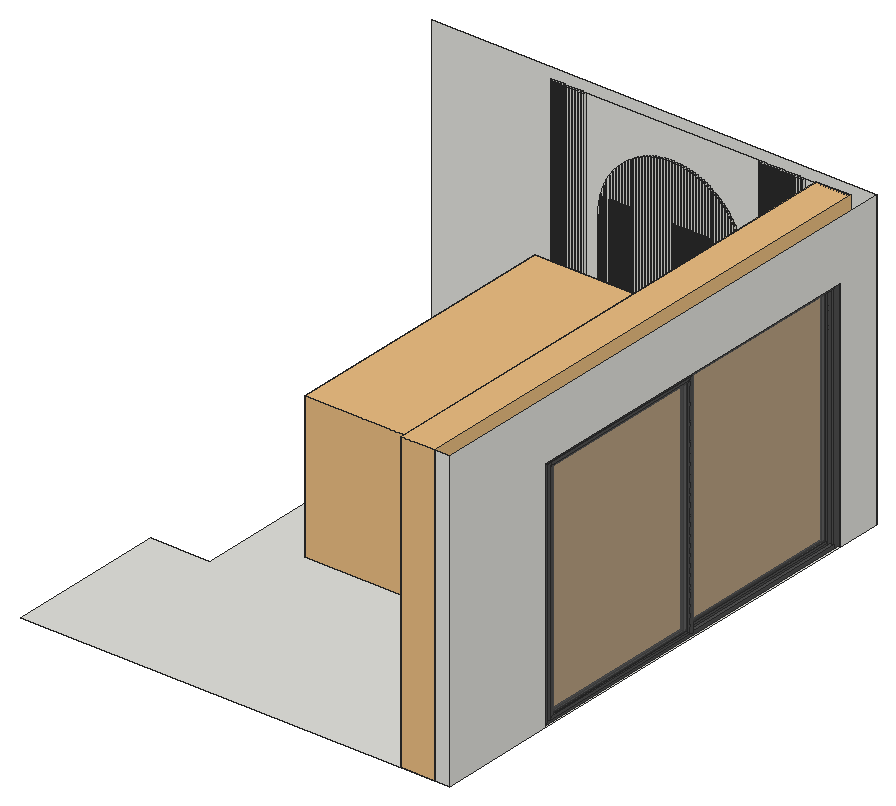
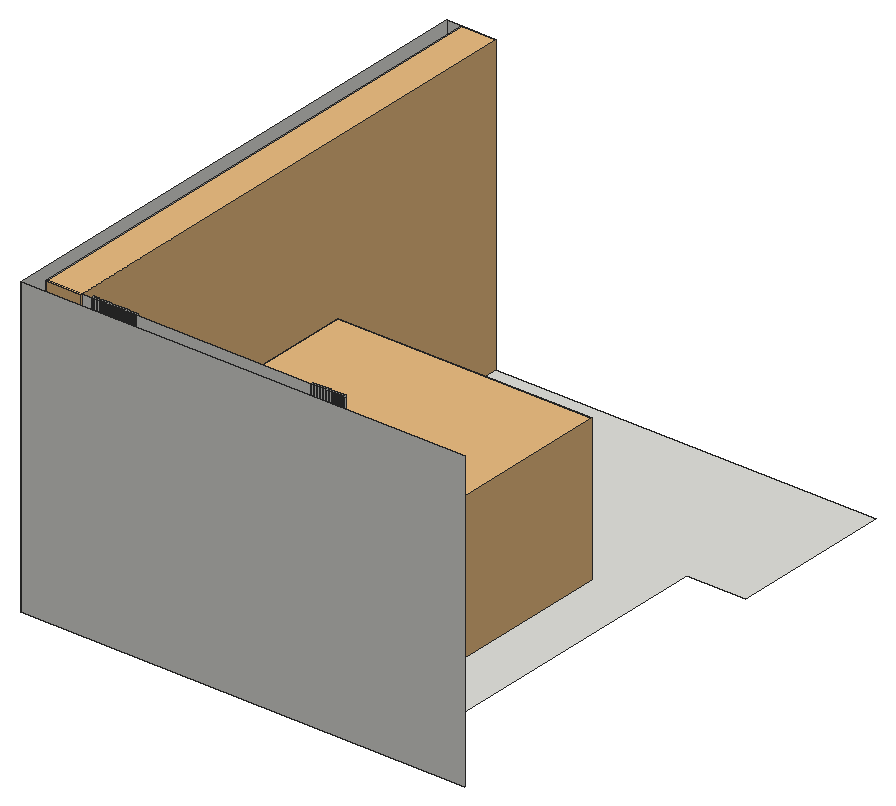
# SketchUp Ruby script. Lengths in inches.
U = 1.inch
M = Sketchup.active_model
def pt(a) = Geom::Point3d.new(a.map { |v| v * U })
def face(e, loops, mat)
  f = e.add_face(loops[0].map { |a| pt(a) })
  loops[1..].each { |l| e.add_face(l.map { |a| pt(a) }).erase! }
  f.material = f.back_material = mat if mat
  f
end
# faces: each face lists its corners as indices into pts; further lists are holes
def faces(e, pts, list, mat = nil) = list.each { |f| face(e, (f[0].is_a?(Array) ? f : [f]).map { |l| l.map { |i| pts[i] } }, mat) }
# xy, xz, yz: faces in a plane at the given z, y or x. An outline is a flat list of corners, or four numbers for a rectangle; further outlines are holes
def ring(l) = l.size == 4 ? [[l[0], l[1]], [l[2], l[1]], [l[2], l[3]], [l[0], l[3]]] : l.each_slice(2).to_a
def flat(e, list, mat, &to3) = list.each { |f| face(e, (f[0].is_a?(Array) ? f : [f]).map { |l| ring(l).map { |u, v| to3.(u, v) } }, mat) }
def xy(e, z, list, mat = nil) = flat(e, list, mat) { |x, y| [x, y, z] }
def xz(e, y, list, mat = nil) = flat(e, list, mat) { |x, z| [x, y, z] }
def yz(e, x, list, mat = nil) = flat(e, list, mat) { |y, z| [x, y, z] }
def lines(e, pts, list) = list.each { |a, b| e.add_line(pt(pts[a]), pt(pts[b])) }
# prism: a flat outline (further loops are holes) pulled along v
def prism(e, loops, v, mat = nil)
  f = face(e, loops, mat); d = Geom::Vector3d.new(v.map { |x| x * U })
  f.pushpull(f.normal.samedirection?(d) ? d.length : -d.length)
end
def box(e, o, s, mat = nil) = prism(e, [[o, [o[0] + s[0], o[1], o[2]], [o[0] + s[0], o[1] + s[1], o[2]], [o[0], o[1] + s[1], o[2]]]], [0, 0, s[2]], mat)
def at(x, y, z, deg = 0) = Geom::Transformation.translation(pt([x, y, z])) * Geom::Transformation.rotation(ORIGIN, Z_AXIS, deg.degrees)
def axes(o, x, y, z) = Geom::Transformation.new([*x, 0, *y, 0, *z, 0, *pt(o).to_a, 1])
def part(name) = M.definitions.add(name)
# library, detail: a bought-in or finely detailed component or shape, given as its bounding box
def library(name, o, s) = part(name).tap { |d| box(d.entities, o, s) }
def detail(e, o, s) = box(e.add_group.entities, o, s)
def put(e, d, t, mat = nil) = e.add_instance(d, t).tap { |i| i.material = mat if mat }
def group(e, t, mat = nil) = e.add_group.tap { |g| g.transformation = t; g.material = mat if mat }.entities
root = M.entities
M.materials.add("[0135_DarkGray]").color = [81, 81, 81]
M.materials.add("[Translucent Glass Gray]").color = [128, 128, 128]
M.materials["[Translucent Glass Gray]"].alpha = 0.15
c1 = library("Bed",[-100.55,9.74,0],[90.43,103.1,58.68])
c2 = library("Curtains with rod \#1",[2.63,-1.46,0.02],[153.32,14.02,114.15])
c3 = part("PENTEK_RP Fineline 50S_Sliding_DoorCase_E1")
box(c3.entities,[0,0,0],[1.51,3.66,99.27],"[0135_DarkGray]")
c4 = part("PENTEK_RP Fineline 50S_SlidingDooe_Case_E2")
box(c4.entities,[0,0,0],[96.25,3.66,1.51],"[0135_DarkGray]")
c5 = part("pentek_RP Fineline 50S_SlidingDoor_Case")
put(c5.entities,c3,at(97.76,0,0))
put(c5.entities,c4,at(1.51,0,0))
put(c5.entities,c3,at(0,0,0))
put(c5.entities,c4,at(1.51,0,97.76))
c6 = part("PENTEK_RP Fineline 50S_SlidingDoor_GlazingBead_2")
box(c6.entities,[0,0,0],[0.56,0.59,94.39],"[0135_DarkGray]")
c7 = part("PENTEK_RP Fineline 50S_SlidingDoor_Glass")
box(c7.entities,[0,0,0],[46.58,0.16,94.39],"[Translucent Glass Gray]")
c8 = part("PENTEK_RP Fineline 50S_SlidingDoor_GlazingBead")
box(c8.entities,[0,0,0],[45.47,0.59,0.56],"[0135_DarkGray]")
c9 = part("PENTEK_RP Fineline 50S_SlidingDoor_Leaf_E1")
xy(c9.entities,0,[[0,0,0.93,1.97],[0.93,1.57,1.49,1.97]],"[0135_DarkGray]")
xy(c9.entities,96.25,[[0,0,0.93,0,0.93,1.57,1.49,1.57,1.49,1.97,0,1.97]],"[0135_DarkGray]")
xz(c9.entities,0,[[0,0,0.93,96.25]],"[0135_DarkGray]")
xz(c9.entities,1.57,[[0.93,0,1.49,95.32],[0.93,95.32,1.49,96.25]],"[0135_DarkGray]")
xz(c9.entities,1.97,[[0,0,1.49,96.25]],"[0135_DarkGray]")
yz(c9.entities,0,[[0,0,1.97,96.25]],"[0135_DarkGray]")
yz(c9.entities,0.93,[[0,0,1.57,0.93],[0,0.93,1.57,95.32],[0,95.32,1.57,96.25]],"[0135_DarkGray]")
yz(c9.entities,1.49,[[1.57,0,1.97,95.32],[1.57,95.32,1.97,96.25]],"[0135_DarkGray]")
c10 = part("PENTEK_RP Fineline 50S_SlidingDoor_Leaf_E2")
xy(c10.entities,0,[[0,0,0,1.57,0.56,1.57,0.56,1.97,46.02,1.97,46.02,1.57,46.58,1.57,46.58,0]],"[0135_DarkGray]")
xy(c10.entities,0.93,[[0,0,46.58,1.57]],"[0135_DarkGray]")
xy(c10.entities,1.49,[[0.56,1.57,46.02,1.97]],"[0135_DarkGray]")
xz(c10.entities,0,[[0,0,46.58,0.93]],"[0135_DarkGray]")
xz(c10.entities,1.57,[[0,0,0.56,0.93],[46.02,0,46.58,0.93],[0.56,0.93,46.02,1.49]],"[0135_DarkGray]")
xz(c10.entities,1.97,[[0.56,0,46.02,1.49]],"[0135_DarkGray]")
yz(c10.entities,0,[[0,0,1.57,0.93]],"[0135_DarkGray]")
yz(c10.entities,0.56,[[1.57,0,1.97,0.93],[1.57,0.93,1.97,1.49]],"[0135_DarkGray]")
yz(c10.entities,46.02,[[1.57,0,1.97,0.93],[1.57,0.93,1.97,1.49]],"[0135_DarkGray]")
yz(c10.entities,46.58,[[0,0,1.57,0.93]],"[0135_DarkGray]")
c11 = part("PENTEK_RP Fineline S_SlidingDoor_Leaf1")
put(c11.entities,c6,at(0.93,0,0.93))
put(c11.entities,c6,at(46.96,0,0.93))
put(c11.entities,c7,at(1.49,1.42,0.93))
put(c11.entities,c8,at(1.49,0,0.93))
put(c11.entities,c7,at(1.49,0.59,0.93))
put(c11.entities,c9,at(0,0,0))
put(c11.entities,c9,axes([48.44,0,0],[-1,0,0],[0,1,0],[0,0,1]))
put(c11.entities,c10,axes([0.93,0,96.25],[1,0,0],[0,1,0],[0,0,-1]))
put(c11.entities,c10,at(0.93,0,0))
put(c11.entities,c8,at(1.49,0,94.77))
c12 = part("PENTEK_RP Fineline 50S_SlidingDoor_Leaf2")
put(c12.entities,c7,at(1.49,1.42,0.93))
put(c12.entities,c8,at(1.49,0,94.77))
put(c12.entities,c6,at(46.96,0,0.93))
put(c12.entities,c7,at(1.49,0.59,0.93))
put(c12.entities,c6,at(0.93,0,0.93))
put(c12.entities,c9,at(0,0,0))
put(c12.entities,c9,axes([48.44,0,0],[-1,0,0],[0,1,0],[0,0,1]))
put(c12.entities,c8,at(1.49,0,0.93))
put(c12.entities,c10,axes([0.93,0,96.25],[1,0,0],[0,1,0],[0,0,-1]))
put(c12.entities,c10,at(0.93,0,0))
xy(root,0,[[245.003,0,413.003,0,413.003,48,419.003,48,419.003,198,413.003,198,413.003,210,269.003,210,269.003,66,245.003,66]])
xy(root,1,[[315.353,208.6875,316.353,210],[369.353,208.875,370.353,210],[370.553,208.875,371.003,210],[293.003,209,294.003,210],[294.203,209,295.203,210],
  [295.403,209,296.403,210],[296.603,209,297.603,210],[297.803,209,298.803,210],[299.003,209,300.003,210],[300.203,209,301.203,210],
  [301.403,209,302.403,210],[302.603,209,303.603,210],[303.803,209,304.803,210],[305.003,209,306.003,210],[311.79,209,312.753,210],
  [312.953,209,313.953,210],[314.153,209,315.153,210],[316.553,209,317.553,210],[317.753,209,318.753,210],[318.953,209,319.953,210],
  [320.153,209,321.153,210],[321.353,209,322.353,210],[322.553,209,323.553,210],[323.753,209,324.753,210],[324.953,209,325.953,210],
  [326.153,209,327.153,210],[327.353,209,328.353,210],[328.553,209,329.553,210],[329.753,209,330.753,210],[330.953,209,331.953,210],
  [332.153,209,333.153,210],[333.353,209,334.353,210],[334.553,209,335.553,210],[335.753,209,336.753,210],[336.953,209,337.953,210],
  [338.153,209,339.153,210],[339.353,209,340.353,210],[340.553,209,341.553,210],[341.753,209,342.753,210],[342.953,209,343.953,210],
  [344.153,209,345.153,210],[345.353,209,346.353,210],[346.553,209,347.553,210],[347.753,209,348.753,210],[348.953,209,349.953,210],
  [350.153,209,351.153,210],[351.353,209,352.353,210],[352.553,209,353.553,210],[353.753,209,354.753,210],[354.953,209,355.953,210],
  [356.153,209,357.153,210],[357.353,209,358.353,210],[358.553,209,359.553,210],[359.753,209,360.753,210],[360.953,209,361.953,210],
  [362.153,209,363.153,210],[363.353,209,364.353,210],[364.553,209,365.553,210],[365.753,209,366.753,210],[366.953,209,367.953,210],
  [368.153,209,369.153,210],[377.003,209,378.003,210],[378.203,209,379.203,210],[379.403,209,380.403,210],[380.603,209,381.603,210],
  [381.803,209,382.803,210],[383.003,209,384.003,210],[384.203,209,385.203,210],[385.403,209,386.403,210],[386.603,209,387.603,210],
  [387.803,209,388.803,210],[389.003,209,390.166,210],[390.366,209,391.366,210],[391.566,209,392.728,210],[392.928,209,393.928,210],
  [394.128,209,395.003,210]])
xz(root,0,[[413.003,0,419.003,120]])
xz(root,48,[[413.003,0,419.003,96]])
xz(root,198,[[413.003,0,419.003,96]])
xz(root,208.6875,[[315.353,1,316.353,1,316.353,93.787,316.153,93.469,315.756,92.803,315.378,92.127,315.353,92.08]])
xz(root,208.875,[[369.353,1,370.353,1,370.353,84.169,370.185,84.912,369.994,85.663,369.784,86.409,369.554,87.149,369.353,87.741],[370.553,1,371.003,1,371.003,78,370.993,78.775,370.962,79.549,370.912,80.323,370.841,81.095,370.75,81.864,370.639,82.631,370.553,83.129]])
xz(root,209,[[293.003,1,294.003,120],[294.203,1,295.203,120],[295.403,1,296.403,120],[296.603,1,297.603,120],[297.803,1,298.803,120],
  [299.003,1,300.003,120],[300.203,1,301.203,120],[301.403,1,302.403,120],[302.603,1,303.603,120],[303.803,1,304.803,120],
  [305.003,1,306.003,120],[311.79,1,312.753,1,312.753,85.483,312.608,84.912,312.437,84.156,312.286,83.395,312.154,82.631,312.043,81.864,311.952,81.095,311.881,80.323,311.83,79.549,311.8,78.775,311.79,78],[312.953,1,313.953,1,313.953,89.103,313.756,88.61,313.488,87.883,313.239,87.149,313.009,86.409,312.953,86.21],[314.153,1,315.153,1,315.153,91.7,315.017,91.441,314.674,90.746,314.349,90.042,314.153,89.585],[316.553,1,317.553,1,317.553,95.548,317.444,95.402,316.997,94.769,316.566,94.125,316.553,94.104],
  [317.753,1,318.753,1,318.753,97.071,318.388,96.632,317.908,96.023,317.753,95.816],[318.953,1,319.953,1,319.953,98.413,319.921,98.38,319.394,97.811,318.953,97.307],[320.153,1,321.153,1,321.153,99.602,321.017,99.476,320.461,98.935,320.153,98.619],[321.353,1,322.353,1,322.353,100.667,322.168,100.513,321.586,100.002,321.353,99.787],[322.553,1,323.553,1,323.553,101.623,323.373,101.489,322.764,101.009,322.553,100.833],
  [323.753,1,324.753,1,324.753,102.484,324.627,102.4,323.994,101.952,323.753,101.772],[324.953,1,325.953,1,325.953,103.259,325.927,103.244,325.271,102.83,324.953,102.617],[326.153,1,327.153,1,327.153,103.954,326.593,103.64,326.153,103.378],[327.353,1,328.353,1,328.353,104.576,327.955,104.38,327.353,104.063],[328.553,1,329.553,1,329.553,105.132,329.354,105.047,328.65,104.723,328.553,104.675],
  [329.753,1,330.753,1,330.753,105.627,330.066,105.353,329.753,105.218],[330.953,1,331.953,1,331.953,106.058,331.514,105.908,330.953,105.702],[332.153,1,333.153,1,333.153,106.434,332.988,106.387,332.247,106.158,332.153,106.126],[333.353,1,334.353,1,334.353,106.755,333.734,106.598,333.353,106.49],[334.553,1,335.553,1,335.553,107.022,335.241,106.96,334.553,106.804],
  [335.753,1,336.753,1,336.753,107.24,336.001,107.111,335.753,107.062],[336.953,1,337.953,1,337.953,107.403,337.532,107.353,336.953,107.269],[338.153,1,339.153,1,339.153,107.521,339.073,107.515,338.302,107.444,338.153,107.427],[339.353,1,340.353,1,340.353,107.586,339.847,107.566,339.353,107.534],[340.553,1,341.553,1,341.553,107.605,341.396,107.607,340.621,107.596,340.553,107.594],
  [341.753,1,342.753,1,342.753,107.574,342.171,107.596,341.753,107.602],[342.953,1,343.953,1,343.953,107.494,343.719,107.515,342.953,107.566],[344.153,1,345.153,1,345.153,107.366,344.491,107.444,344.153,107.476],[345.353,1,346.353,1,346.353,107.186,346.028,107.242,345.353,107.34],[346.553,1,347.553,1,347.553,106.959,347.552,106.96,346.792,107.111,346.553,107.152],
  [347.753,1,348.753,1,348.753,106.676,348.308,106.789,347.753,106.914],[348.953,1,349.953,1,349.953,106.342,349.805,106.387,349.059,106.598,348.953,106.625],[350.153,1,351.153,1,351.153,105.951,350.545,106.158,350.153,106.279],[351.353,1,352.353,1,352.353,105.502,352.006,105.64,351.353,105.881],[352.553,1,353.553,1,353.553,104.994,353.439,105.047,352.726,105.353,352.553,105.422],
  [353.753,1,354.753,1,354.753,104.421,354.142,104.723,353.753,104.902],[354.953,1,355.953,1,355.953,103.778,355.523,104.019,354.953,104.319],[356.153,1,357.153,1,357.153,103.0625,356.866,103.244,356.2,103.64,356.153,103.666],[357.353,1,358.353,1,358.353,102.267,358.166,102.4,357.521,102.83,357.353,102.936],[358.553,1,359.553,1,359.553,101.383,359.42,101.489,358.799,101.952,358.553,102.126],
  [359.753,1,360.753,1,360.753,100.4,360.624,100.513,360.028,101.009,359.753,101.226],[360.953,1,361.953,1,361.953,99.304,361.776,99.476,361.207,100.002,360.953,100.225],[362.153,1,363.153,1,363.153,98.076,362.872,98.38,362.331,98.935,362.153,99.109],[363.353,1,364.353,1,364.353,96.695,363.909,97.228,363.398,97.811,363.353,97.86],[364.553,1,365.553,1,365.553,95.113,365.349,95.402,364.885,96.023,364.553,96.444],
  [365.753,1,366.753,1,366.753,93.28,366.64,93.469,366.227,94.125,365.796,94.769,365.753,94.83],[366.953,1,367.953,1,367.953,91.082,367.776,91.441,367.415,92.127,367.037,92.803,366.953,92.944],[368.153,1,369.153,1,369.153,88.294,369.037,88.61,368.749,89.33,368.443,90.042,368.153,90.672],[377.003,1,378.003,120],[378.203,1,379.203,120],
  [379.403,1,380.403,120],[380.603,1,381.603,120],[381.803,1,382.803,120],[383.003,1,384.003,120],[384.203,1,385.203,120],
  [385.403,1,386.403,120],[386.603,1,387.603,120],[387.803,1,388.803,120],[389.003,1,390.166,120],[390.366,1,391.366,120],
  [391.566,1,392.728,120],[392.928,1,393.928,120],[394.128,1,395.003,120]])
xz(root,210,[[287.003,0,305.003,1],[305.003,0,311.79,1],[311.79,0,312.79,1],[312.79,0,371.003,1],[371.003,0,377.003,1],
  [377.003,0,395.003,1],[395.003,0,413.003,120],[291.803,1,292.803,120],[292.803,1,293.003,120],[293.003,1,294.003,120],
  [294.003,1,294.203,120],[294.203,1,295.203,120],[295.203,1,295.403,120],[295.403,1,296.403,120],[296.403,1,296.603,120],
  [296.603,1,297.603,120],[297.603,1,297.803,120],[297.803,1,298.803,120],[298.803,1,299.003,120],[299.003,1,300.003,120],
  [300.003,1,300.203,120],[300.203,1,301.203,120],[301.203,1,301.403,120],[301.403,1,302.403,120],[302.403,1,302.603,120],
  [302.603,1,303.603,120],[303.603,1,303.803,120],[303.803,1,304.803,120],[304.803,1,305.003,120],[305.003,1,306.003,120],
  [306.003,1,311.79,1,311.79,78,311.8,78.775,311.83,79.549,311.881,80.323,311.952,81.095,312.043,81.864,312.154,82.631,312.286,83.395,312.437,84.156,312.608,84.912,312.753,85.483,312.79,85.628,312.799,85.663,312.953,86.21,313.009,86.409,313.239,87.149,313.488,87.883,313.756,88.61,313.953,89.103,313.99,89.195,314.043,89.33,314.153,89.585,314.349,90.042,314.674,90.746,315.017,91.441,315.153,91.7,315.353,92.08,315.378,92.127,315.756,92.803,316.153,93.469,316.353,93.787,316.553,94.104,316.566,94.125,316.997,94.769,317.444,95.402,317.553,95.548,317.753,95.816,317.908,96.023,318.388,96.632,318.753,97.071,318.883,97.228,318.953,97.307,319.394,97.811,319.921,98.38,319.953,98.413,320.153,98.619,320.461,98.935,321.017,99.476,321.153,99.602,321.353,99.787,321.586,100.002,322.168,100.513,322.353,100.667,322.553,100.833,322.764,101.009,323.373,101.489,323.553,101.623,323.753,101.772,323.994,101.952,324.627,102.4,324.753,102.484,324.953,102.617,325.271,102.83,325.927,103.244,325.953,103.259,326.153,103.378,326.593,103.64,327.153,103.954,327.269,104.019,327.353,104.063,327.955,104.38,328.353,104.576,328.553,104.675,328.65,104.723,329.354,105.047,329.553,105.132,329.753,105.218,330.066,105.353,330.753,105.627,330.786,105.64,330.953,105.702,331.514,105.908,331.953,106.058,332.153,106.126,332.247,106.158,332.988,106.387,333.153,106.434,333.353,106.49,333.734,106.598,334.353,106.755,334.485,106.789,334.553,106.804,335.241,106.96,335.553,107.022,335.753,107.062,336.001,107.111,336.753,107.24,336.765,107.242,336.953,107.269,337.532,107.353,337.953,107.403,338.153,107.427,338.302,107.444,339.073,107.515,339.153,107.521,339.353,107.534,339.847,107.566,340.353,107.586,340.553,107.594,340.621,107.596,341.396,107.607,341.553,107.605,341.753,107.602,342.171,107.596,342.753,107.574,342.946,107.566,342.953,107.566,343.719,107.515,343.953,107.494,344.153,107.476,344.491,107.444,345.153,107.366,345.261,107.353,345.353,107.34,346.028,107.242,346.353,107.186,346.553,107.152,346.792,107.111,347.552,106.96,347.553,106.959,347.753,106.914,348.308,106.789,348.753,106.676,348.953,106.625,349.059,106.598,349.805,106.387,349.953,106.342,350.153,106.279,350.545,106.158,351.153,105.951,351.279,105.908,351.353,105.881,352.006,105.64,352.353,105.502,352.553,105.422,352.726,105.353,353.439,105.047,353.553,104.994,353.753,104.902,354.142,104.723,354.753,104.421,354.838,104.38,354.953,104.319,355.523,104.019,355.953,103.778,356.153,103.666,356.2,103.64,356.866,103.244,357.153,103.0625,357.353,102.936,357.521,102.83,358.166,102.4,358.353,102.267,358.553,102.126,358.799,101.952,359.42,101.489,359.553,101.383,359.753,101.226,360.028,101.009,360.624,100.513,360.753,100.4,360.953,100.225,361.207,100.002,361.776,99.476,361.953,99.304,362.153,99.109,362.331,98.935,362.872,98.38,363.153,98.076,363.353,97.86,363.398,97.811,363.909,97.228,364.353,96.695,364.405,96.632,364.553,96.444,364.885,96.023,365.349,95.402,365.553,95.113,365.753,94.83,365.796,94.769,366.227,94.125,366.64,93.469,366.753,93.28,366.953,92.944,367.037,92.803,367.415,92.127,367.776,91.441,367.953,91.082,368.119,90.746,368.153,90.672,368.443,90.042,368.749,89.33,369.037,88.61,369.153,88.294,369.305,87.883,369.353,87.741,369.554,87.149,369.784,86.409,369.994,85.663,370.185,84.912,370.353,84.169,370.356,84.156,370.507,83.395,370.553,83.129,370.639,82.631,370.75,81.864,370.841,81.095,370.912,80.323,370.962,79.549,370.993,78.775,371.003,78,371.003,1,377.003,1,377.003,120,306.003,120],[312.753,1,312.79,1,312.79,85.628,312.753,85.483],[312.79,1,312.953,1,312.953,86.21,312.799,85.663,312.79,85.628],[313.953,1,314.153,1,314.153,89.585,314.043,89.33,313.99,89.195,313.953,89.103],[315.153,1,315.353,1,315.353,92.08,315.153,91.7],
  [316.353,1,316.553,1,316.553,94.104,316.353,93.787],[317.553,1,317.753,1,317.753,95.816,317.553,95.548],[318.753,1,318.953,1,318.953,97.307,318.883,97.228,318.753,97.071],[319.953,1,320.153,1,320.153,98.619,319.953,98.413],[321.153,1,321.353,1,321.353,99.787,321.153,99.602],
  [322.353,1,322.553,1,322.553,100.833,322.353,100.667],[323.553,1,323.753,1,323.753,101.772,323.553,101.623],[324.753,1,324.953,1,324.953,102.617,324.753,102.484],[325.953,1,326.153,1,326.153,103.378,325.953,103.259],[327.153,1,327.353,1,327.353,104.063,327.269,104.019,327.153,103.954],
  [328.353,1,328.553,1,328.553,104.675,328.353,104.576],[329.553,1,329.753,1,329.753,105.218,329.553,105.132],[330.753,1,330.953,1,330.953,105.702,330.786,105.64,330.753,105.627],[331.953,1,332.153,1,332.153,106.126,331.953,106.058],[333.153,1,333.353,1,333.353,106.49,333.153,106.434],
  [334.353,1,334.553,1,334.553,106.804,334.485,106.789,334.353,106.755],[335.553,1,335.753,1,335.753,107.062,335.553,107.022],[336.753,1,336.953,1,336.953,107.269,336.765,107.242,336.753,107.24],[337.953,1,338.153,1,338.153,107.427,337.953,107.403],[339.153,1,339.353,1,339.353,107.534,339.153,107.521],
  [340.353,1,340.553,1,340.553,107.594,340.353,107.586],[341.553,1,341.753,1,341.753,107.602,341.553,107.605],[342.753,1,342.953,1,342.953,107.566,342.946,107.566,342.753,107.574],[343.953,1,344.153,1,344.153,107.476,343.953,107.494],[345.153,1,345.353,1,345.353,107.34,345.261,107.353,345.153,107.366],
  [346.353,1,346.553,1,346.553,107.152,346.353,107.186],[347.553,1,347.753,1,347.753,106.914,347.553,106.959],[348.753,1,348.953,1,348.953,106.625,348.753,106.676],[349.953,1,350.153,1,350.153,106.279,349.953,106.342],[351.153,1,351.353,1,351.353,105.881,351.279,105.908,351.153,105.951],
  [352.353,1,352.553,1,352.553,105.422,352.353,105.502],[353.553,1,353.753,1,353.753,104.902,353.553,104.994],[354.753,1,354.953,1,354.953,104.319,354.838,104.38,354.753,104.421],[355.953,1,356.153,1,356.153,103.666,355.953,103.778],[357.153,1,357.353,1,357.353,102.936,357.153,103.0625],
  [358.353,1,358.553,1,358.553,102.126,358.353,102.267],[359.553,1,359.753,1,359.753,101.226,359.553,101.383],[360.753,1,360.953,1,360.953,100.225,360.753,100.4],[361.953,1,362.153,1,362.153,99.109,361.953,99.304],[363.153,1,363.353,1,363.353,97.86,363.153,98.076],
  [364.353,1,364.553,1,364.553,96.444,364.405,96.632,364.353,96.695],[365.553,1,365.753,1,365.753,94.83,365.553,95.113],[366.753,1,366.953,1,366.953,92.944,366.753,93.28],[367.953,1,368.153,1,368.153,90.672,368.119,90.746,367.953,91.082],[369.153,1,369.353,1,369.353,87.741,369.305,87.883,369.153,88.294],
  [370.353,1,370.553,1,370.553,83.129,370.507,83.395,370.356,84.156,370.353,84.169],[377.003,1,378.003,120],[378.003,1,378.203,120],[378.203,1,379.203,120],[379.203,1,379.403,120],
  [379.403,1,380.403,120],[380.403,1,380.603,120],[380.603,1,381.603,120],[381.603,1,381.803,120],[381.803,1,382.803,120],
  [382.803,1,383.003,120],[383.003,1,384.003,120],[384.003,1,384.203,120],[384.203,1,385.203,120],[385.203,1,385.403,120],
  [385.403,1,386.403,120],[386.403,1,386.603,120],[386.603,1,387.603,120],[387.603,1,387.803,120],[387.803,1,388.803,120],
  [388.803,1,389.003,120],[389.003,1,390.166,120],[390.166,1,390.366,120],[390.366,1,391.366,120],[391.366,1,391.566,120],
  [391.566,1,392.728,120],[392.728,1,392.928,120],[392.928,1,393.928,120],[393.928,1,394.128,120],[394.128,1,395.003,120]])
xz(root,216,[[239.003,0,419.003,120]])
yz(root,292.803,[[209,1,210,120]])
yz(root,293.003,[[209,1,210,120]])
yz(root,294.003,[[209,1,210,120]])
yz(root,294.203,[[209,1,210,120]])
yz(root,295.203,[[209,1,210,120]])
yz(root,295.403,[[209,1,210,120]])
yz(root,296.403,[[209,1,210,120]])
yz(root,296.603,[[209,1,210,120]])
yz(root,297.603,[[209,1,210,120]])
yz(root,297.803,[[209,1,210,120]])
yz(root,298.803,[[209,1,210,120]])
yz(root,299.003,[[209,1,210,120]])
yz(root,300.003,[[209,1,210,120]])
yz(root,300.203,[[209,1,210,120]])
yz(root,301.203,[[209,1,210,120]])
yz(root,301.403,[[209,1,210,120]])
yz(root,302.403,[[209,1,210,120]])
yz(root,302.603,[[209,1,210,120]])
yz(root,303.603,[[209,1,210,120]])
yz(root,303.803,[[209,1,210,120]])
yz(root,304.803,[[209,1,210,120]])
yz(root,305.003,[[209,1,210,120]])
yz(root,306.003,[[209,1,210,120]])
yz(root,311.79,[[209,1,210,78]])
yz(root,312.753,[[209,1,210,85.483]])
yz(root,312.953,[[209,1,210,86.21]])
yz(root,313.953,[[209,1,210,85.483]])
yz(root,314.153,[[209,1,210,89.585]])
yz(root,315.153,[[209,1,210,85.483]])
yz(root,315.353,[[208.6875,1,210,92.08]])
yz(root,316.353,[[208.6875,1,210,85.483]])
yz(root,316.553,[[209,1,210,94.104]])
yz(root,317.553,[[209,1,210,85.483]])
yz(root,317.753,[[209,1,210,95.816]])
yz(root,318.753,[[209,1,210,85.483]])
yz(root,318.953,[[209,1,210,97.307]])
yz(root,319.953,[[209,1,210,85.483]])
yz(root,320.153,[[209,1,210,98.619]])
yz(root,321.153,[[209,1,210,85.483]])
yz(root,321.353,[[209,1,210,99.787]])
yz(root,322.353,[[209,1,210,85.483]])
yz(root,322.553,[[209,1,210,100.833]])
yz(root,323.553,[[209,1,210,85.483]])
yz(root,323.753,[[209,1,210,101.772]])
yz(root,324.753,[[209,1,210,85.483]])
yz(root,324.953,[[209,1,210,102.617]])
yz(root,325.953,[[209,1,210,85.483]])
yz(root,326.153,[[209,1,210,103.378]])
yz(root,327.153,[[209,1,210,85.483]])
yz(root,327.353,[[209,1,210,104.063]])
yz(root,328.353,[[209,1,210,85.483]])
yz(root,328.553,[[209,1,210,104.675]])
yz(root,329.553,[[209,1,210,85.483]])
yz(root,329.753,[[209,1,210,105.218]])
yz(root,330.753,[[209,1,210,85.483]])
yz(root,330.953,[[209,1,210,105.702]])
yz(root,331.953,[[209,1,210,85.483]])
yz(root,332.153,[[209,1,210,106.126]])
yz(root,333.153,[[209,1,210,85.483]])
yz(root,333.353,[[209,1,210,106.49]])
yz(root,334.353,[[209,1,210,85.483]])
yz(root,334.553,[[209,1,210,106.804]])
yz(root,335.553,[[209,1,210,85.483]])
yz(root,335.753,[[209,1,210,107.062]])
yz(root,336.753,[[209,1,210,85.483]])
yz(root,336.953,[[209,1,210,107.269]])
yz(root,337.953,[[209,1,210,85.483]])
yz(root,338.153,[[209,1,210,107.427]])
yz(root,339.153,[[209,1,210,85.483]])
yz(root,339.353,[[209,1,210,107.534]])
yz(root,340.353,[[209,1,210,85.483]])
yz(root,340.553,[[209,1,210,107.594]])
yz(root,341.553,[[209,1,210,85.483]])
yz(root,341.753,[[209,1,210,107.602]])
yz(root,342.753,[[209,1,210,85.483]])
yz(root,342.953,[[209,1,210,107.566]])
yz(root,343.953,[[209,1,210,85.483]])
yz(root,344.153,[[209,1,210,107.476]])
yz(root,345.153,[[209,1,210,85.483]])
yz(root,345.353,[[209,1,210,107.34]])
yz(root,346.353,[[209,1,210,85.483]])
yz(root,346.553,[[209,1,210,107.152]])
yz(root,347.553,[[209,1,210,85.483]])
yz(root,347.753,[[209,1,210,106.914]])
yz(root,348.753,[[209,1,210,85.483]])
yz(root,348.953,[[209,1,210,106.625]])
yz(root,349.953,[[209,1,210,85.483]])
yz(root,350.153,[[209,1,210,106.279]])
yz(root,351.153,[[209,1,210,85.483]])
yz(root,351.353,[[209,1,210,105.881]])
yz(root,352.353,[[209,1,210,85.483]])
yz(root,352.553,[[209,1,210,105.422]])
yz(root,353.553,[[209,1,210,85.483]])
yz(root,353.753,[[209,1,210,104.902]])
yz(root,354.753,[[209,1,210,85.483]])
yz(root,354.953,[[209,1,210,104.319]])
yz(root,355.953,[[209,1,210,85.483]])
yz(root,356.153,[[209,1,210,103.666]])
yz(root,357.153,[[209,1,210,85.483]])
yz(root,357.353,[[209,1,210,102.936]])
yz(root,358.353,[[209,1,210,85.483]])
yz(root,358.553,[[209,1,210,102.126]])
yz(root,359.553,[[209,1,210,85.483]])
yz(root,359.753,[[209,1,210,101.226]])
yz(root,360.753,[[209,1,210,85.483]])
yz(root,360.953,[[209,1,210,100.225]])
yz(root,361.953,[[209,1,210,85.483]])
yz(root,362.153,[[209,1,210,99.109]])
yz(root,363.153,[[209,1,210,85.483]])
yz(root,363.353,[[209,1,210,97.86]])
yz(root,364.353,[[209,1,210,85.483]])
yz(root,364.553,[[209,1,210,96.444]])
yz(root,365.553,[[209,1,210,85.483]])
yz(root,365.753,[[209,1,210,94.83]])
yz(root,366.753,[[209,1,210,85.483]])
yz(root,366.953,[[209,1,210,92.944]])
yz(root,367.953,[[209,1,210,85.483]])
yz(root,368.153,[[209,1,210,90.672]])
yz(root,369.153,[[209,1,210,85.483]])
yz(root,369.353,[[208.875,1,210,87.741]])
yz(root,370.353,[[208.875,1,210,84.169]])
yz(root,370.553,[[208.875,1,210,83.129]])
yz(root,371.003,[[208.875,1,210,78]])
yz(root,377.003,[[209,1,210,120]])
yz(root,378.003,[[209,1,210,120]])
yz(root,378.203,[[209,1,210,120]])
yz(root,379.203,[[209,1,210,120]])
yz(root,379.403,[[209,1,210,120]])
yz(root,380.403,[[209,1,210,120]])
yz(root,380.603,[[209,1,210,120]])
yz(root,381.603,[[209,1,210,120]])
yz(root,381.803,[[209,1,210,120]])
yz(root,382.803,[[209,1,210,120]])
yz(root,383.003,[[209,1,210,120]])
yz(root,384.003,[[209,1,210,120]])
yz(root,384.203,[[209,1,210,120]])
yz(root,385.203,[[209,1,210,120]])
yz(root,385.403,[[209,1,210,120]])
yz(root,386.403,[[209,1,210,120]])
yz(root,386.603,[[209,1,210,120]])
yz(root,387.603,[[209,1,210,120]])
yz(root,387.803,[[209,1,210,120]])
yz(root,388.803,[[209,1,210,120]])
yz(root,389.003,[[209,1,210,120]])
yz(root,390.166,[[209,1,210,120]])
yz(root,390.366,[[209,1,210,120]])
yz(root,391.366,[[209,1,210,120]])
yz(root,391.566,[[209,1,210,120]])
yz(root,392.728,[[209,1,210,120]])
yz(root,392.928,[[209,1,210,120]])
yz(root,393.928,[[209,1,210,120]])
yz(root,394.128,[[209,1,210,120]])
yz(root,395.003,[[209,1,210,120]])
yz(root,413.003,[[0,0,0,120,210,120,210,0,198,0,198,96,48,96,48,0]])
yz(root,419.003,[[0,0,48,0,48,96,198,96,198,0,216,0,216,120,0,120]])
put(root,c1,axes([280.99,73.6875,0],[0,-1.29,0],[1,0,0],[0,0,1]))
put(root,c2,axes([400.45,214.15,-0.02],[0,-1.37316,0],[1,0,0],[0,0,1.0512]))
g1 = group(root,at(414.51,48,0))
put(g1,c5,axes([3.66,0,0],[0,1.511,0],[-1,0,0],[0,0,0.96704]))
put(g1,c11,axes([4.06,2.28,1.46],[0,1.511,0],[-1,0,0],[0,0,0.96704]))
put(g1,c12,axes([2.09,74.52,1.46],[0,1.511,0],[-1,0,0],[0,0,0.96704]))
